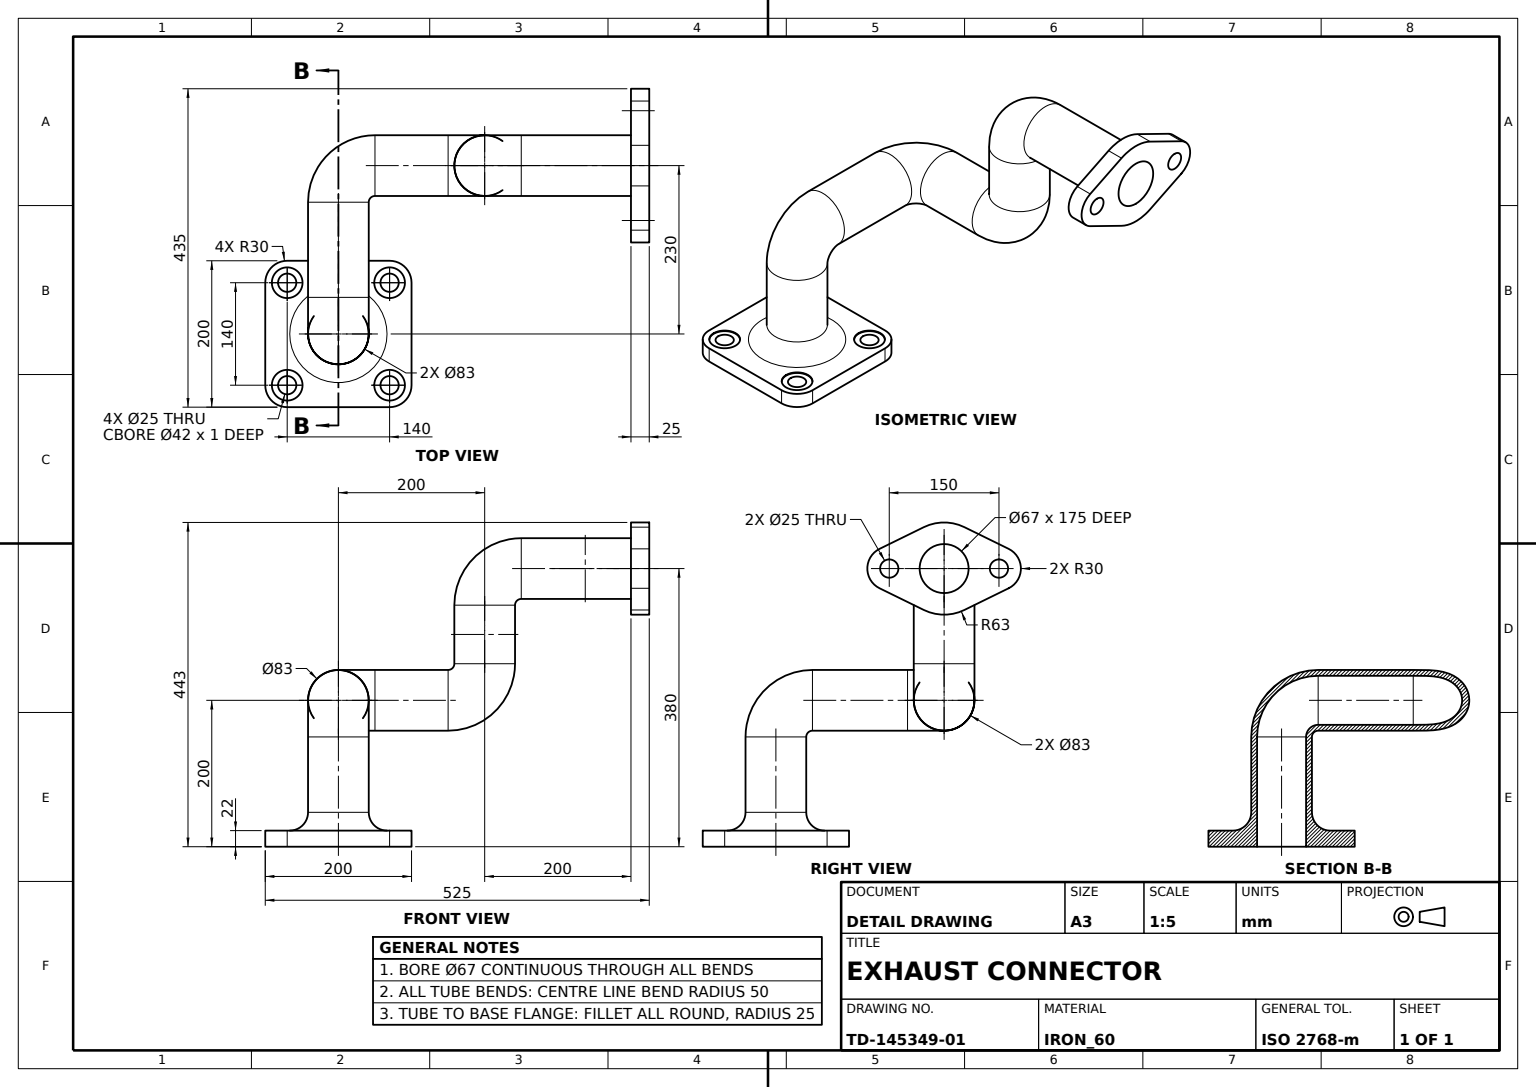
ISO-10303-21;
HEADER;
FILE_DESCRIPTION((''),'2;1');
FILE_NAME('','',(''),(''),'','','');
FILE_SCHEMA(('AUTOMOTIVE_DESIGN'));
ENDSEC;
DATA;
#1=APPLICATION_CONTEXT('');
#2=PRODUCT_CONTEXT('',#1,'mechanical');
#3=PRODUCT('','','',(#2));
#4=PRODUCT_DEFINITION_FORMATION('','',#3);
#5=PRODUCT_DEFINITION_CONTEXT('',#1,'design');
#6=PRODUCT_DEFINITION('','',#4,#5);
#7=PRODUCT_DEFINITION_SHAPE('','',#6);
#8=(LENGTH_UNIT()NAMED_UNIT(*)SI_UNIT(.MILLI.,.METRE.));
#9=(NAMED_UNIT(*)PLANE_ANGLE_UNIT()SI_UNIT($,.RADIAN.));
#10=(NAMED_UNIT(*)SI_UNIT($,.STERADIAN.)SOLID_ANGLE_UNIT());
#11=UNCERTAINTY_MEASURE_WITH_UNIT(LENGTH_MEASURE(0.005),#8,'distance_accuracy_value','');
#12=(GEOMETRIC_REPRESENTATION_CONTEXT(3)GLOBAL_UNCERTAINTY_ASSIGNED_CONTEXT((#11))GLOBAL_UNIT_ASSIGNED_CONTEXT((#8,#9,#10))REPRESENTATION_CONTEXT('',''));
#13=CARTESIAN_POINT('',(400.,202.28,323.42614));
#14=VERTEX_POINT('',#13);
#15=CARTESIAN_POINT('',(400.,257.72,323.42614));
#16=VERTEX_POINT('',#15);
#17=CARTESIAN_POINT('',(400.,230.,380.));
#18=DIRECTION('',(1.,0.,0.));
#19=DIRECTION('',(0.,1.,0.));
#20=AXIS2_PLACEMENT_3D('',#17,#18,#19);
#21=CIRCLE('',#20,63.);
#22=EDGE_CURVE('',#14,#16,#21,.T.);
#23=ORIENTED_EDGE('',*,*,#22,.T.);
#24=CARTESIAN_POINT('',(425.,257.72,323.42614));
#25=VERTEX_POINT('',#24);
#26=VECTOR('',#18,1000.);
#27=LINE('',#15,#26);
#28=EDGE_CURVE('',#16,#25,#27,.T.);
#29=ORIENTED_EDGE('',*,*,#28,.T.);
#30=CARTESIAN_POINT('',(425.,202.28,323.42614));
#31=VERTEX_POINT('',#30);
#32=CARTESIAN_POINT('',(425.,230.,380.));
#33=AXIS2_PLACEMENT_3D('',#32,#18,#19);
#34=CIRCLE('',#33,63.);
#35=EDGE_CURVE('',#31,#25,#34,.T.);
#36=ORIENTED_EDGE('',*,*,#35,.F.);
#37=LINE('',#13,#26);
#38=EDGE_CURVE('',#14,#31,#37,.T.);
#39=ORIENTED_EDGE('',*,*,#38,.F.);
#40=EDGE_LOOP('',(#23,#29,#36,#39));
#41=FACE_BOUND('',#40,.T.);
#42=DIRECTION('',(0.,0.,-1.));
#43=AXIS2_PLACEMENT_3D('',#17,#18,#42);
#44=CYLINDRICAL_SURFACE('',#43,63.);
#45=ADVANCED_FACE('',(#41),#44,.T.);
#46=CARTESIAN_POINT('',(233.5,230.,330.));
#47=VERTEX_POINT('',#46);
#48=CARTESIAN_POINT('',(200.,230.,330.));
#49=DIRECTION('',(0.,0.,1.));
#50=AXIS2_PLACEMENT_3D('',#48,#49,#18);
#51=CIRCLE('',#50,33.5);
#52=EDGE_CURVE('',#47,#47,#51,.T.);
#53=ORIENTED_EDGE('',*,*,#52,.F.);
#54=EDGE_LOOP('',(#53));
#55=FACE_BOUND('',#54,.T.);
#56=CARTESIAN_POINT('',(250.,230.,346.5));
#57=VERTEX_POINT('',#56);
#58=CARTESIAN_POINT('',(250.,230.,380.));
#59=AXIS2_PLACEMENT_3D('',#58,#18,#42);
#60=CIRCLE('',#59,33.5);
#61=EDGE_CURVE('',#57,#57,#60,.T.);
#62=ORIENTED_EDGE('',*,*,#61,.T.);
#63=EDGE_LOOP('',(#62));
#64=FACE_BOUND('',#63,.T.);
#65=CARTESIAN_POINT('',(250.,230.,330.));
#66=AXIS2_PLACEMENT_3D('',#65,#19,#49);
#67=TOROIDAL_SURFACE('',#66,50.,33.5);
#68=ADVANCED_FACE('',(#55,#64),#67,.F.);
#69=CARTESIAN_POINT('',(-82.5,-70.,21.));
#70=VERTEX_POINT('',#69);
#71=CARTESIAN_POINT('',(-70.,-70.,21.));
#72=DIRECTION('',(-1.,0.,0.));
#73=AXIS2_PLACEMENT_3D('',#71,#42,#72);
#74=CIRCLE('',#73,12.5);
#75=EDGE_CURVE('',#70,#70,#74,.F.);
#76=ORIENTED_EDGE('',*,*,#75,.F.);
#77=EDGE_LOOP('',(#76));
#78=FACE_BOUND('',#77,.T.);
#79=CARTESIAN_POINT('',(-91.,-70.,21.));
#80=VERTEX_POINT('',#79);
#81=CIRCLE('',#73,21.);
#82=EDGE_CURVE('',#80,#80,#81,.F.);
#83=ORIENTED_EDGE('',*,*,#82,.T.);
#84=EDGE_LOOP('',(#83));
#85=FACE_BOUND('',#84,.T.);
#86=PLANE('',#73);
#87=ADVANCED_FACE('',(#78,#85),#86,.F.);
#88=CARTESIAN_POINT('',(49.,70.,22.));
#89=VERTEX_POINT('',#88);
#90=CARTESIAN_POINT('',(70.,70.,22.));
#91=AXIS2_PLACEMENT_3D('',#90,#42,#72);
#92=CIRCLE('',#91,21.);
#93=EDGE_CURVE('',#89,#89,#92,.T.);
#94=ORIENTED_EDGE('',*,*,#93,.T.);
#95=EDGE_LOOP('',(#94));
#96=FACE_BOUND('',#95,.T.);
#97=CARTESIAN_POINT('',(-66.5,0.,22.));
#98=VERTEX_POINT('',#97);
#99=CARTESIAN_POINT('',(0.,0.,22.));
#100=AXIS2_PLACEMENT_3D('',#99,#42,#72);
#101=CIRCLE('',#100,66.5);
#102=EDGE_CURVE('',#98,#98,#101,.T.);
#103=ORIENTED_EDGE('',*,*,#102,.T.);
#104=EDGE_LOOP('',(#103));
#105=FACE_BOUND('',#104,.T.);
#106=CARTESIAN_POINT('',(49.,-70.,22.));
#107=VERTEX_POINT('',#106);
#108=CARTESIAN_POINT('',(70.,-70.,22.));
#109=AXIS2_PLACEMENT_3D('',#108,#42,#72);
#110=CIRCLE('',#109,21.);
#111=EDGE_CURVE('',#107,#107,#110,.T.);
#112=ORIENTED_EDGE('',*,*,#111,.T.);
#113=EDGE_LOOP('',(#112));
#114=FACE_BOUND('',#113,.T.);
#115=CARTESIAN_POINT('',(-91.,70.,22.));
#116=VERTEX_POINT('',#115);
#117=CARTESIAN_POINT('',(-70.,70.,22.));
#118=AXIS2_PLACEMENT_3D('',#117,#42,#72);
#119=CIRCLE('',#118,21.);
#120=EDGE_CURVE('',#116,#116,#119,.T.);
#121=ORIENTED_EDGE('',*,*,#120,.T.);
#122=EDGE_LOOP('',(#121));
#123=FACE_BOUND('',#122,.T.);
#124=CARTESIAN_POINT('',(100.,70.,22.));
#125=VERTEX_POINT('',#124);
#126=CARTESIAN_POINT('',(100.,-70.,22.));
#127=VERTEX_POINT('',#126);
#128=CARTESIAN_POINT('',(100.,100.,22.));
#129=DIRECTION('',(0.,-1.,0.));
#130=VECTOR('',#129,1000.);
#131=LINE('',#128,#130);
#132=EDGE_CURVE('',#125,#127,#131,.T.);
#133=ORIENTED_EDGE('',*,*,#132,.F.);
#134=CARTESIAN_POINT('',(70.,100.,22.));
#135=VERTEX_POINT('',#134);
#136=CIRCLE('',#91,30.);
#137=EDGE_CURVE('',#125,#135,#136,.F.);
#138=ORIENTED_EDGE('',*,*,#137,.T.);
#139=CARTESIAN_POINT('',(-70.,100.,22.));
#140=VERTEX_POINT('',#139);
#141=CARTESIAN_POINT('',(-100.,100.,22.));
#142=LINE('',#141,#26);
#143=EDGE_CURVE('',#140,#135,#142,.T.);
#144=ORIENTED_EDGE('',*,*,#143,.F.);
#145=CARTESIAN_POINT('',(-100.,70.,22.));
#146=VERTEX_POINT('',#145);
#147=CIRCLE('',#118,30.);
#148=EDGE_CURVE('',#140,#146,#147,.F.);
#149=ORIENTED_EDGE('',*,*,#148,.T.);
#150=CARTESIAN_POINT('',(-100.,-70.,22.));
#151=VERTEX_POINT('',#150);
#152=CARTESIAN_POINT('',(-100.,-100.,22.));
#153=VECTOR('',#19,1000.);
#154=LINE('',#152,#153);
#155=EDGE_CURVE('',#151,#146,#154,.T.);
#156=ORIENTED_EDGE('',*,*,#155,.F.);
#157=CARTESIAN_POINT('',(-70.,-100.,22.));
#158=VERTEX_POINT('',#157);
#159=CARTESIAN_POINT('',(-70.,-70.,22.));
#160=AXIS2_PLACEMENT_3D('',#159,#42,#72);
#161=CIRCLE('',#160,30.);
#162=EDGE_CURVE('',#151,#158,#161,.F.);
#163=ORIENTED_EDGE('',*,*,#162,.T.);
#164=CARTESIAN_POINT('',(70.,-100.,22.));
#165=VERTEX_POINT('',#164);
#166=CARTESIAN_POINT('',(100.,-100.,22.));
#167=VECTOR('',#72,1000.);
#168=LINE('',#166,#167);
#169=EDGE_CURVE('',#165,#158,#168,.T.);
#170=ORIENTED_EDGE('',*,*,#169,.F.);
#171=CIRCLE('',#109,30.);
#172=EDGE_CURVE('',#165,#127,#171,.F.);
#173=ORIENTED_EDGE('',*,*,#172,.T.);
#174=EDGE_LOOP('',(#133,#138,#144,#149,#156,#163,#170,#173));
#175=FACE_BOUND('',#174,.T.);
#176=CARTESIAN_POINT('',(-91.,-70.,22.));
#177=VERTEX_POINT('',#176);
#178=CIRCLE('',#160,21.);
#179=EDGE_CURVE('',#177,#177,#178,.T.);
#180=ORIENTED_EDGE('',*,*,#179,.T.);
#181=EDGE_LOOP('',(#180));
#182=FACE_BOUND('',#181,.T.);
#183=PLANE('',#100);
#184=ADVANCED_FACE('',(#96,#105,#114,#123,#175,#182),#183,.F.);
#185=CARTESIAN_POINT('',(400.,141.8,406.939933));
#186=VERTEX_POINT('',#185);
#187=CARTESIAN_POINT('',(400.,141.8,353.060067));
#188=VERTEX_POINT('',#187);
#189=CARTESIAN_POINT('',(400.,155.,380.));
#190=AXIS2_PLACEMENT_3D('',#189,#18,#19);
#191=CIRCLE('',#190,30.);
#192=EDGE_CURVE('',#186,#188,#191,.T.);
#193=ORIENTED_EDGE('',*,*,#192,.T.);
#194=CARTESIAN_POINT('',(425.,141.8,353.060067));
#195=VERTEX_POINT('',#194);
#196=LINE('',#187,#26);
#197=EDGE_CURVE('',#188,#195,#196,.T.);
#198=ORIENTED_EDGE('',*,*,#197,.T.);
#199=CARTESIAN_POINT('',(425.,141.8,406.939933));
#200=VERTEX_POINT('',#199);
#201=CARTESIAN_POINT('',(425.,155.,380.));
#202=AXIS2_PLACEMENT_3D('',#201,#18,#19);
#203=CIRCLE('',#202,30.);
#204=EDGE_CURVE('',#200,#195,#203,.T.);
#205=ORIENTED_EDGE('',*,*,#204,.F.);
#206=LINE('',#185,#26);
#207=EDGE_CURVE('',#186,#200,#206,.T.);
#208=ORIENTED_EDGE('',*,*,#207,.F.);
#209=EDGE_LOOP('',(#193,#198,#205,#208));
#210=FACE_BOUND('',#209,.T.);
#211=AXIS2_PLACEMENT_3D('',#189,#18,#42);
#212=CYLINDRICAL_SURFACE('',#211,30.);
#213=ADVANCED_FACE('',(#210),#212,.T.);
#214=CARTESIAN_POINT('',(425.,230.,413.5));
#215=VERTEX_POINT('',#214);
#216=AXIS2_PLACEMENT_3D('',#32,#72,#49);
#217=CIRCLE('',#216,33.5);
#218=EDGE_CURVE('',#215,#215,#217,.T.);
#219=ORIENTED_EDGE('',*,*,#218,.F.);
#220=EDGE_LOOP('',(#219));
#221=FACE_BOUND('',#220,.T.);
#222=ORIENTED_EDGE('',*,*,#61,.F.);
#223=EDGE_LOOP('',(#222));
#224=FACE_BOUND('',#223,.T.);
#225=CYLINDRICAL_SURFACE('',#59,33.5);
#226=ADVANCED_FACE('',(#221,#224),#225,.F.);
#227=CARTESIAN_POINT('',(49.,70.,21.));
#228=VERTEX_POINT('',#227);
#229=CARTESIAN_POINT('',(70.,70.,21.));
#230=AXIS2_PLACEMENT_3D('',#229,#42,#72);
#231=CIRCLE('',#230,21.);
#232=EDGE_CURVE('',#228,#228,#231,.F.);
#233=ORIENTED_EDGE('',*,*,#232,.F.);
#234=EDGE_LOOP('',(#233));
#235=FACE_BOUND('',#234,.T.);
#236=ORIENTED_EDGE('',*,*,#93,.F.);
#237=EDGE_LOOP('',(#236));
#238=FACE_BOUND('',#237,.T.);
#239=CYLINDRICAL_SURFACE('',#91,21.);
#240=ADVANCED_FACE('',(#235,#238),#239,.F.);
#241=CARTESIAN_POINT('',(425.,155.,392.5));
#242=VERTEX_POINT('',#241);
#243=AXIS2_PLACEMENT_3D('',#201,#72,#49);
#244=CIRCLE('',#243,12.5);
#245=EDGE_CURVE('',#242,#242,#244,.T.);
#246=ORIENTED_EDGE('',*,*,#245,.T.);
#247=EDGE_LOOP('',(#246));
#248=FACE_BOUND('',#247,.T.);
#249=CARTESIAN_POINT('',(425.,305.,392.5));
#250=VERTEX_POINT('',#249);
#251=CARTESIAN_POINT('',(425.,305.,380.));
#252=AXIS2_PLACEMENT_3D('',#251,#72,#49);
#253=CIRCLE('',#252,12.5);
#254=EDGE_CURVE('',#250,#250,#253,.T.);
#255=ORIENTED_EDGE('',*,*,#254,.T.);
#256=EDGE_LOOP('',(#255));
#257=FACE_BOUND('',#256,.T.);
#258=ORIENTED_EDGE('',*,*,#218,.T.);
#259=EDGE_LOOP('',(#258));
#260=FACE_BOUND('',#259,.T.);
#261=CARTESIAN_POINT('',(425.,318.2,353.060067));
#262=VERTEX_POINT('',#261);
#263=CARTESIAN_POINT('',(425.,318.2,406.939933));
#264=VERTEX_POINT('',#263);
#265=AXIS2_PLACEMENT_3D('',#251,#18,#19);
#266=CIRCLE('',#265,30.);
#267=EDGE_CURVE('',#262,#264,#266,.T.);
#268=ORIENTED_EDGE('',*,*,#267,.T.);
#269=CARTESIAN_POINT('',(425.,257.72,436.57386));
#270=VERTEX_POINT('',#269);
#271=DIRECTION('',(0.,-0.897997773,0.44));
#272=VECTOR('',#271,1000.);
#273=LINE('',#263,#272);
#274=EDGE_CURVE('',#264,#270,#273,.T.);
#275=ORIENTED_EDGE('',*,*,#274,.T.);
#276=CARTESIAN_POINT('',(425.,202.28,436.57386));
#277=VERTEX_POINT('',#276);
#278=EDGE_CURVE('',#270,#277,#34,.T.);
#279=ORIENTED_EDGE('',*,*,#278,.T.);
#280=DIRECTION('',(0.,-0.897997773,-0.44));
#281=VECTOR('',#280,1000.);
#282=LINE('',#276,#281);
#283=EDGE_CURVE('',#277,#200,#282,.T.);
#284=ORIENTED_EDGE('',*,*,#283,.T.);
#285=ORIENTED_EDGE('',*,*,#204,.T.);
#286=DIRECTION('',(0.,0.897997773,-0.44));
#287=VECTOR('',#286,1000.);
#288=LINE('',#194,#287);
#289=EDGE_CURVE('',#195,#31,#288,.T.);
#290=ORIENTED_EDGE('',*,*,#289,.T.);
#291=ORIENTED_EDGE('',*,*,#35,.T.);
#292=DIRECTION('',(0.,0.897997773,0.44));
#293=VECTOR('',#292,1000.);
#294=LINE('',#24,#293);
#295=EDGE_CURVE('',#25,#262,#294,.T.);
#296=ORIENTED_EDGE('',*,*,#295,.T.);
#297=EDGE_LOOP('',(#268,#275,#279,#284,#285,#290,#291,#296));
#298=FACE_BOUND('',#297,.T.);
#299=AXIS2_PLACEMENT_3D('',#251,#18,#42);
#300=PLANE('',#299);
#301=ADVANCED_FACE('',(#248,#257,#260,#298),#300,.T.);
#302=ORIENTED_EDGE('',*,*,#155,.T.);
#303=CARTESIAN_POINT('',(-100.,70.,0.));
#304=VERTEX_POINT('',#303);
#305=VECTOR('',#42,1000.);
#306=LINE('',#145,#305);
#307=EDGE_CURVE('',#146,#304,#306,.T.);
#308=ORIENTED_EDGE('',*,*,#307,.T.);
#309=CARTESIAN_POINT('',(-100.,-70.,0.));
#310=VERTEX_POINT('',#309);
#311=CARTESIAN_POINT('',(-100.,-100.,0.));
#312=LINE('',#311,#153);
#313=EDGE_CURVE('',#310,#304,#312,.T.);
#314=ORIENTED_EDGE('',*,*,#313,.F.);
#315=LINE('',#150,#305);
#316=EDGE_CURVE('',#310,#151,#315,.F.);
#317=ORIENTED_EDGE('',*,*,#316,.T.);
#318=EDGE_LOOP('',(#302,#308,#314,#317));
#319=FACE_BOUND('',#318,.T.);
#320=AXIS2_PLACEMENT_3D('',#152,#72,#49);
#321=PLANE('',#320);
#322=ADVANCED_FACE('',(#319),#321,.T.);
#323=CARTESIAN_POINT('',(233.5,230.,250.));
#324=VERTEX_POINT('',#323);
#325=CARTESIAN_POINT('',(200.,230.,250.));
#326=AXIS2_PLACEMENT_3D('',#325,#49,#18);
#327=CIRCLE('',#326,33.5);
#328=EDGE_CURVE('',#324,#324,#327,.T.);
#329=ORIENTED_EDGE('',*,*,#328,.T.);
#330=EDGE_LOOP('',(#329));
#331=FACE_BOUND('',#330,.T.);
#332=CARTESIAN_POINT('',(150.,230.,166.5));
#333=VERTEX_POINT('',#332);
#334=CARTESIAN_POINT('',(150.,230.,200.));
#335=AXIS2_PLACEMENT_3D('',#334,#18,#42);
#336=CIRCLE('',#335,33.5);
#337=EDGE_CURVE('',#333,#333,#336,.T.);
#338=ORIENTED_EDGE('',*,*,#337,.F.);
#339=EDGE_LOOP('',(#338));
#340=FACE_BOUND('',#339,.T.);
#341=CARTESIAN_POINT('',(150.,230.,250.));
#342=AXIS2_PLACEMENT_3D('',#341,#129,#42);
#343=TOROIDAL_SURFACE('',#342,50.,33.5);
#344=ADVANCED_FACE('',(#331,#340),#343,.F.);
#345=CARTESIAN_POINT('',(0.,180.,158.5));
#346=VERTEX_POINT('',#345);
#347=CARTESIAN_POINT('',(0.,180.,200.));
#348=AXIS2_PLACEMENT_3D('',#347,#129,#42);
#349=CIRCLE('',#348,41.5);
#350=EDGE_CURVE('',#346,#346,#349,.T.);
#351=ORIENTED_EDGE('',*,*,#350,.F.);
#352=EDGE_LOOP('',(#351));
#353=FACE_BOUND('',#352,.T.);
#354=CARTESIAN_POINT('',(50.,271.5,200.));
#355=VERTEX_POINT('',#354);
#356=CARTESIAN_POINT('',(50.,230.,200.));
#357=AXIS2_PLACEMENT_3D('',#356,#18,#19);
#358=CIRCLE('',#357,41.5);
#359=EDGE_CURVE('',#355,#355,#358,.T.);
#360=ORIENTED_EDGE('',*,*,#359,.F.);
#361=EDGE_LOOP('',(#360));
#362=FACE_BOUND('',#361,.T.);
#363=CARTESIAN_POINT('',(50.,180.,200.));
#364=AXIS2_PLACEMENT_3D('',#363,#42,#72);
#365=TOROIDAL_SURFACE('',#364,50.,41.5);
#366=ADVANCED_FACE('',(#353,#362),#365,.T.);
#367=CARTESIAN_POINT('',(-70.,100.,0.));
#368=VERTEX_POINT('',#367);
#369=CARTESIAN_POINT('',(-70.,70.,0.));
#370=AXIS2_PLACEMENT_3D('',#369,#42,#72);
#371=CIRCLE('',#370,30.);
#372=EDGE_CURVE('',#304,#368,#371,.T.);
#373=ORIENTED_EDGE('',*,*,#372,.F.);
#374=ORIENTED_EDGE('',*,*,#307,.F.);
#375=ORIENTED_EDGE('',*,*,#148,.F.);
#376=LINE('',#139,#305);
#377=EDGE_CURVE('',#368,#140,#376,.F.);
#378=ORIENTED_EDGE('',*,*,#377,.F.);
#379=EDGE_LOOP('',(#373,#374,#375,#378));
#380=FACE_BOUND('',#379,.T.);
#381=CYLINDRICAL_SURFACE('',#118,30.);
#382=ADVANCED_FACE('',(#380),#381,.T.);
#383=ORIENTED_EDGE('',*,*,#350,.T.);
#384=EDGE_LOOP('',(#383));
#385=FACE_BOUND('',#384,.T.);
#386=CARTESIAN_POINT('',(0.,50.,158.5));
#387=VERTEX_POINT('',#386);
#388=CARTESIAN_POINT('',(0.,50.,200.));
#389=AXIS2_PLACEMENT_3D('',#388,#129,#42);
#390=CIRCLE('',#389,41.5);
#391=EDGE_CURVE('',#387,#387,#390,.T.);
#392=ORIENTED_EDGE('',*,*,#391,.F.);
#393=EDGE_LOOP('',(#392));
#394=FACE_BOUND('',#393,.T.);
#395=AXIS2_PLACEMENT_3D('',#388,#19,#49);
#396=CYLINDRICAL_SURFACE('',#395,41.5);
#397=ADVANCED_FACE('',(#385,#394),#396,.T.);
#398=CARTESIAN_POINT('',(50.,263.5,200.));
#399=VERTEX_POINT('',#398);
#400=CIRCLE('',#357,33.5);
#401=EDGE_CURVE('',#399,#399,#400,.T.);
#402=ORIENTED_EDGE('',*,*,#401,.F.);
#403=EDGE_LOOP('',(#402));
#404=FACE_BOUND('',#403,.T.);
#405=ORIENTED_EDGE('',*,*,#337,.T.);
#406=EDGE_LOOP('',(#405));
#407=FACE_BOUND('',#406,.T.);
#408=AXIS2_PLACEMENT_3D('',#356,#18,#42);
#409=CYLINDRICAL_SURFACE('',#408,33.5);
#410=ADVANCED_FACE('',(#404,#407),#409,.F.);
#411=CARTESIAN_POINT('',(-82.5,-70.,0.));
#412=VERTEX_POINT('',#411);
#413=CARTESIAN_POINT('',(-70.,-70.,0.));
#414=AXIS2_PLACEMENT_3D('',#413,#42,#72);
#415=CIRCLE('',#414,12.5);
#416=EDGE_CURVE('',#412,#412,#415,.T.);
#417=ORIENTED_EDGE('',*,*,#416,.T.);
#418=EDGE_LOOP('',(#417));
#419=FACE_BOUND('',#418,.T.);
#420=ORIENTED_EDGE('',*,*,#75,.T.);
#421=EDGE_LOOP('',(#420));
#422=FACE_BOUND('',#421,.T.);
#423=CARTESIAN_POINT('',(-70.,-70.,-28.));
#424=AXIS2_PLACEMENT_3D('',#423,#42,#72);
#425=CYLINDRICAL_SURFACE('',#424,12.5);
#426=ADVANCED_FACE('',(#419,#422),#425,.F.);
#427=CARTESIAN_POINT('',(0.,180.,166.5));
#428=VERTEX_POINT('',#427);
#429=CIRCLE('',#348,33.5);
#430=EDGE_CURVE('',#428,#428,#429,.T.);
#431=ORIENTED_EDGE('',*,*,#430,.T.);
#432=EDGE_LOOP('',(#431));
#433=FACE_BOUND('',#432,.T.);
#434=ORIENTED_EDGE('',*,*,#401,.T.);
#435=EDGE_LOOP('',(#434));
#436=FACE_BOUND('',#435,.T.);
#437=TOROIDAL_SURFACE('',#364,50.,33.5);
#438=ADVANCED_FACE('',(#433,#436),#437,.F.);
#439=CARTESIAN_POINT('',(250.,230.,338.5));
#440=VERTEX_POINT('',#439);
#441=CIRCLE('',#59,41.5);
#442=EDGE_CURVE('',#440,#440,#441,.T.);
#443=ORIENTED_EDGE('',*,*,#442,.T.);
#444=EDGE_LOOP('',(#443));
#445=FACE_BOUND('',#444,.T.);
#446=CARTESIAN_POINT('',(400.,230.,338.5));
#447=VERTEX_POINT('',#446);
#448=CIRCLE('',#43,41.5);
#449=EDGE_CURVE('',#447,#447,#448,.T.);
#450=ORIENTED_EDGE('',*,*,#449,.F.);
#451=EDGE_LOOP('',(#450));
#452=FACE_BOUND('',#451,.T.);
#453=CYLINDRICAL_SURFACE('',#59,41.5);
#454=ADVANCED_FACE('',(#445,#452),#453,.T.);
#455=ORIENTED_EDGE('',*,*,#278,.F.);
#456=CARTESIAN_POINT('',(400.,257.72,436.57386));
#457=VERTEX_POINT('',#456);
#458=LINE('',#456,#26);
#459=EDGE_CURVE('',#457,#270,#458,.T.);
#460=ORIENTED_EDGE('',*,*,#459,.F.);
#461=CARTESIAN_POINT('',(400.,202.28,436.57386));
#462=VERTEX_POINT('',#461);
#463=EDGE_CURVE('',#457,#462,#21,.T.);
#464=ORIENTED_EDGE('',*,*,#463,.T.);
#465=LINE('',#461,#26);
#466=EDGE_CURVE('',#462,#277,#465,.T.);
#467=ORIENTED_EDGE('',*,*,#466,.T.);
#468=EDGE_LOOP('',(#455,#460,#464,#467));
#469=FACE_BOUND('',#468,.T.);
#470=ADVANCED_FACE('',(#469),#44,.T.);
#471=ORIENTED_EDGE('',*,*,#102,.F.);
#472=EDGE_LOOP('',(#471));
#473=FACE_BOUND('',#472,.T.);
#474=CARTESIAN_POINT('',(-41.5,0.,47.));
#475=VERTEX_POINT('',#474);
#476=CARTESIAN_POINT('',(0.,0.,47.));
#477=AXIS2_PLACEMENT_3D('',#476,#42,#72);
#478=CIRCLE('',#477,41.5);
#479=EDGE_CURVE('',#475,#475,#478,.F.);
#480=ORIENTED_EDGE('',*,*,#479,.F.);
#481=EDGE_LOOP('',(#480));
#482=FACE_BOUND('',#481,.T.);
#483=TOROIDAL_SURFACE('',#477,66.5,25.);
#484=ADVANCED_FACE('',(#473,#482),#483,.F.);
#485=ORIENTED_EDGE('',*,*,#479,.T.);
#486=EDGE_LOOP('',(#485));
#487=FACE_BOUND('',#486,.T.);
#488=CARTESIAN_POINT('',(0.,41.5,150.));
#489=VERTEX_POINT('',#488);
#490=CARTESIAN_POINT('',(0.,0.,150.));
#491=AXIS2_PLACEMENT_3D('',#490,#42,#19);
#492=CIRCLE('',#491,41.5);
#493=EDGE_CURVE('',#489,#489,#492,.T.);
#494=ORIENTED_EDGE('',*,*,#493,.T.);
#495=EDGE_LOOP('',(#494));
#496=FACE_BOUND('',#495,.T.);
#497=CYLINDRICAL_SURFACE('',#491,41.5);
#498=ADVANCED_FACE('',(#487,#496),#497,.T.);
#499=ORIENTED_EDGE('',*,*,#493,.F.);
#500=EDGE_LOOP('',(#499));
#501=FACE_BOUND('',#500,.T.);
#502=ORIENTED_EDGE('',*,*,#391,.T.);
#503=EDGE_LOOP('',(#502));
#504=FACE_BOUND('',#503,.T.);
#505=CARTESIAN_POINT('',(0.,50.,150.));
#506=AXIS2_PLACEMENT_3D('',#505,#18,#42);
#507=TOROIDAL_SURFACE('',#506,50.,41.5);
#508=ADVANCED_FACE('',(#501,#504),#507,.T.);
#509=ORIENTED_EDGE('',*,*,#232,.T.);
#510=EDGE_LOOP('',(#509));
#511=FACE_BOUND('',#510,.T.);
#512=CARTESIAN_POINT('',(57.5,70.,21.));
#513=VERTEX_POINT('',#512);
#514=CIRCLE('',#230,12.5);
#515=EDGE_CURVE('',#513,#513,#514,.F.);
#516=ORIENTED_EDGE('',*,*,#515,.F.);
#517=EDGE_LOOP('',(#516));
#518=FACE_BOUND('',#517,.T.);
#519=PLANE('',#230);
#520=ADVANCED_FACE('',(#511,#518),#519,.F.);
#521=ORIENTED_EDGE('',*,*,#283,.F.);
#522=ORIENTED_EDGE('',*,*,#466,.F.);
#523=LINE('',#461,#281);
#524=EDGE_CURVE('',#462,#186,#523,.T.);
#525=ORIENTED_EDGE('',*,*,#524,.T.);
#526=ORIENTED_EDGE('',*,*,#207,.T.);
#527=EDGE_LOOP('',(#521,#522,#525,#526));
#528=FACE_BOUND('',#527,.T.);
#529=DIRECTION('',(0.,-0.44,0.897997773));
#530=AXIS2_PLACEMENT_3D('',#461,#529,#280);
#531=PLANE('',#530);
#532=ADVANCED_FACE('',(#528),#531,.T.);
#533=ORIENTED_EDGE('',*,*,#111,.F.);
#534=EDGE_LOOP('',(#533));
#535=FACE_BOUND('',#534,.T.);
#536=CARTESIAN_POINT('',(49.,-70.,21.));
#537=VERTEX_POINT('',#536);
#538=CARTESIAN_POINT('',(70.,-70.,21.));
#539=AXIS2_PLACEMENT_3D('',#538,#42,#72);
#540=CIRCLE('',#539,21.);
#541=EDGE_CURVE('',#537,#537,#540,.F.);
#542=ORIENTED_EDGE('',*,*,#541,.F.);
#543=EDGE_LOOP('',(#542));
#544=FACE_BOUND('',#543,.T.);
#545=CYLINDRICAL_SURFACE('',#109,21.);
#546=ADVANCED_FACE('',(#535,#544),#545,.F.);
#547=CARTESIAN_POINT('',(0.,33.5,150.));
#548=VERTEX_POINT('',#547);
#549=CIRCLE('',#491,33.5);
#550=EDGE_CURVE('',#548,#548,#549,.T.);
#551=ORIENTED_EDGE('',*,*,#550,.F.);
#552=EDGE_LOOP('',(#551));
#553=FACE_BOUND('',#552,.T.);
#554=CARTESIAN_POINT('',(33.5,0.,0.));
#555=VERTEX_POINT('',#554);
#556=CARTESIAN_POINT('',(0.,0.,0.));
#557=AXIS2_PLACEMENT_3D('',#556,#49,#18);
#558=CIRCLE('',#557,33.5);
#559=EDGE_CURVE('',#555,#555,#558,.T.);
#560=ORIENTED_EDGE('',*,*,#559,.F.);
#561=EDGE_LOOP('',(#560));
#562=FACE_BOUND('',#561,.T.);
#563=CYLINDRICAL_SURFACE('',#491,33.5);
#564=ADVANCED_FACE('',(#553,#562),#563,.F.);
#565=CARTESIAN_POINT('',(0.,50.,166.5));
#566=VERTEX_POINT('',#565);
#567=CIRCLE('',#389,33.5);
#568=EDGE_CURVE('',#566,#566,#567,.T.);
#569=ORIENTED_EDGE('',*,*,#568,.F.);
#570=EDGE_LOOP('',(#569));
#571=FACE_BOUND('',#570,.T.);
#572=ORIENTED_EDGE('',*,*,#550,.T.);
#573=EDGE_LOOP('',(#572));
#574=FACE_BOUND('',#573,.T.);
#575=TOROIDAL_SURFACE('',#506,50.,33.5);
#576=ADVANCED_FACE('',(#571,#574),#575,.F.);
#577=CARTESIAN_POINT('',(150.,230.,158.5));
#578=VERTEX_POINT('',#577);
#579=CIRCLE('',#335,41.5);
#580=EDGE_CURVE('',#578,#578,#579,.T.);
#581=ORIENTED_EDGE('',*,*,#580,.T.);
#582=EDGE_LOOP('',(#581));
#583=FACE_BOUND('',#582,.T.);
#584=CARTESIAN_POINT('',(241.5,230.,250.));
#585=VERTEX_POINT('',#584);
#586=CIRCLE('',#326,41.5);
#587=EDGE_CURVE('',#585,#585,#586,.T.);
#588=ORIENTED_EDGE('',*,*,#587,.F.);
#589=EDGE_LOOP('',(#588));
#590=FACE_BOUND('',#589,.T.);
#591=TOROIDAL_SURFACE('',#342,50.,41.5);
#592=ADVANCED_FACE('',(#583,#590),#591,.T.);
#593=ORIENTED_EDGE('',*,*,#38,.T.);
#594=ORIENTED_EDGE('',*,*,#289,.F.);
#595=ORIENTED_EDGE('',*,*,#197,.F.);
#596=LINE('',#187,#287);
#597=EDGE_CURVE('',#188,#14,#596,.T.);
#598=ORIENTED_EDGE('',*,*,#597,.T.);
#599=EDGE_LOOP('',(#593,#594,#595,#598));
#600=FACE_BOUND('',#599,.T.);
#601=DIRECTION('',(0.,-0.44,-0.897997773));
#602=AXIS2_PLACEMENT_3D('',#187,#601,#286);
#603=PLANE('',#602);
#604=ADVANCED_FACE('',(#600),#603,.T.);
#605=ORIENTED_EDGE('',*,*,#28,.F.);
#606=CARTESIAN_POINT('',(400.,318.2,353.060067));
#607=VERTEX_POINT('',#606);
#608=LINE('',#15,#293);
#609=EDGE_CURVE('',#16,#607,#608,.T.);
#610=ORIENTED_EDGE('',*,*,#609,.T.);
#611=LINE('',#606,#26);
#612=EDGE_CURVE('',#607,#262,#611,.T.);
#613=ORIENTED_EDGE('',*,*,#612,.T.);
#614=ORIENTED_EDGE('',*,*,#295,.F.);
#615=EDGE_LOOP('',(#605,#610,#613,#614));
#616=FACE_BOUND('',#615,.T.);
#617=DIRECTION('',(0.,0.44,-0.897997773));
#618=AXIS2_PLACEMENT_3D('',#15,#617,#292);
#619=PLANE('',#618);
#620=ADVANCED_FACE('',(#616),#619,.T.);
#621=CARTESIAN_POINT('',(70.,-100.,0.));
#622=VERTEX_POINT('',#621);
#623=CARTESIAN_POINT('',(-70.,-100.,0.));
#624=VERTEX_POINT('',#623);
#625=CARTESIAN_POINT('',(100.,-100.,0.));
#626=LINE('',#625,#167);
#627=EDGE_CURVE('',#622,#624,#626,.T.);
#628=ORIENTED_EDGE('',*,*,#627,.T.);
#629=CIRCLE('',#414,30.);
#630=EDGE_CURVE('',#624,#310,#629,.T.);
#631=ORIENTED_EDGE('',*,*,#630,.T.);
#632=ORIENTED_EDGE('',*,*,#313,.T.);
#633=ORIENTED_EDGE('',*,*,#372,.T.);
#634=CARTESIAN_POINT('',(70.,100.,0.));
#635=VERTEX_POINT('',#634);
#636=CARTESIAN_POINT('',(-100.,100.,0.));
#637=LINE('',#636,#26);
#638=EDGE_CURVE('',#368,#635,#637,.T.);
#639=ORIENTED_EDGE('',*,*,#638,.T.);
#640=CARTESIAN_POINT('',(100.,70.,0.));
#641=VERTEX_POINT('',#640);
#642=CARTESIAN_POINT('',(70.,70.,0.));
#643=AXIS2_PLACEMENT_3D('',#642,#42,#72);
#644=CIRCLE('',#643,30.);
#645=EDGE_CURVE('',#635,#641,#644,.T.);
#646=ORIENTED_EDGE('',*,*,#645,.T.);
#647=CARTESIAN_POINT('',(100.,-70.,0.));
#648=VERTEX_POINT('',#647);
#649=CARTESIAN_POINT('',(100.,100.,0.));
#650=LINE('',#649,#130);
#651=EDGE_CURVE('',#641,#648,#650,.T.);
#652=ORIENTED_EDGE('',*,*,#651,.T.);
#653=CARTESIAN_POINT('',(70.,-70.,0.));
#654=AXIS2_PLACEMENT_3D('',#653,#42,#72);
#655=CIRCLE('',#654,30.);
#656=EDGE_CURVE('',#648,#622,#655,.T.);
#657=ORIENTED_EDGE('',*,*,#656,.T.);
#658=EDGE_LOOP('',(#628,#631,#632,#633,#639,#646,#652,#657));
#659=FACE_BOUND('',#658,.T.);
#660=CARTESIAN_POINT('',(57.5,-70.,0.));
#661=VERTEX_POINT('',#660);
#662=CIRCLE('',#654,12.5);
#663=EDGE_CURVE('',#661,#661,#662,.T.);
#664=ORIENTED_EDGE('',*,*,#663,.F.);
#665=EDGE_LOOP('',(#664));
#666=FACE_BOUND('',#665,.T.);
#667=CARTESIAN_POINT('',(57.5,70.,0.));
#668=VERTEX_POINT('',#667);
#669=CIRCLE('',#643,12.5);
#670=EDGE_CURVE('',#668,#668,#669,.T.);
#671=ORIENTED_EDGE('',*,*,#670,.F.);
#672=EDGE_LOOP('',(#671));
#673=FACE_BOUND('',#672,.T.);
#674=ORIENTED_EDGE('',*,*,#559,.T.);
#675=EDGE_LOOP('',(#674));
#676=FACE_BOUND('',#675,.T.);
#677=CARTESIAN_POINT('',(-82.5,70.,0.));
#678=VERTEX_POINT('',#677);
#679=CIRCLE('',#370,12.5);
#680=EDGE_CURVE('',#678,#678,#679,.T.);
#681=ORIENTED_EDGE('',*,*,#680,.F.);
#682=EDGE_LOOP('',(#681));
#683=FACE_BOUND('',#682,.T.);
#684=ORIENTED_EDGE('',*,*,#416,.F.);
#685=EDGE_LOOP('',(#684));
#686=FACE_BOUND('',#685,.T.);
#687=AXIS2_PLACEMENT_3D('',#556,#42,#72);
#688=PLANE('',#687);
#689=ADVANCED_FACE('',(#659,#666,#673,#676,#683,#686),#688,.T.);
#690=CARTESIAN_POINT('',(-91.,70.,21.));
#691=VERTEX_POINT('',#690);
#692=CARTESIAN_POINT('',(-70.,70.,21.));
#693=AXIS2_PLACEMENT_3D('',#692,#42,#72);
#694=CIRCLE('',#693,21.);
#695=EDGE_CURVE('',#691,#691,#694,.F.);
#696=ORIENTED_EDGE('',*,*,#695,.F.);
#697=EDGE_LOOP('',(#696));
#698=FACE_BOUND('',#697,.T.);
#699=ORIENTED_EDGE('',*,*,#120,.F.);
#700=EDGE_LOOP('',(#699));
#701=FACE_BOUND('',#700,.T.);
#702=CYLINDRICAL_SURFACE('',#118,21.);
#703=ADVANCED_FACE('',(#698,#701),#702,.F.);
#704=ORIENTED_EDGE('',*,*,#638,.F.);
#705=ORIENTED_EDGE('',*,*,#377,.T.);
#706=ORIENTED_EDGE('',*,*,#143,.T.);
#707=LINE('',#134,#305);
#708=EDGE_CURVE('',#135,#635,#707,.T.);
#709=ORIENTED_EDGE('',*,*,#708,.T.);
#710=EDGE_LOOP('',(#704,#705,#706,#709));
#711=FACE_BOUND('',#710,.T.);
#712=AXIS2_PLACEMENT_3D('',#141,#19,#49);
#713=PLANE('',#712);
#714=ADVANCED_FACE('',(#711),#713,.T.);
#715=ORIENTED_EDGE('',*,*,#612,.F.);
#716=CARTESIAN_POINT('',(400.,318.2,406.939933));
#717=VERTEX_POINT('',#716);
#718=CARTESIAN_POINT('',(400.,305.,380.));
#719=AXIS2_PLACEMENT_3D('',#718,#18,#19);
#720=CIRCLE('',#719,30.);
#721=EDGE_CURVE('',#607,#717,#720,.T.);
#722=ORIENTED_EDGE('',*,*,#721,.T.);
#723=LINE('',#716,#26);
#724=EDGE_CURVE('',#717,#264,#723,.T.);
#725=ORIENTED_EDGE('',*,*,#724,.T.);
#726=ORIENTED_EDGE('',*,*,#267,.F.);
#727=EDGE_LOOP('',(#715,#722,#725,#726));
#728=FACE_BOUND('',#727,.T.);
#729=AXIS2_PLACEMENT_3D('',#718,#18,#42);
#730=CYLINDRICAL_SURFACE('',#729,30.);
#731=ADVANCED_FACE('',(#728),#730,.T.);
#732=ORIENTED_EDGE('',*,*,#442,.F.);
#733=EDGE_LOOP('',(#732));
#734=FACE_BOUND('',#733,.T.);
#735=CARTESIAN_POINT('',(241.5,230.,330.));
#736=VERTEX_POINT('',#735);
#737=CIRCLE('',#50,41.5);
#738=EDGE_CURVE('',#736,#736,#737,.T.);
#739=ORIENTED_EDGE('',*,*,#738,.T.);
#740=EDGE_LOOP('',(#739));
#741=FACE_BOUND('',#740,.T.);
#742=TOROIDAL_SURFACE('',#66,50.,41.5);
#743=ADVANCED_FACE('',(#734,#741),#742,.T.);
#744=ORIENTED_EDGE('',*,*,#695,.T.);
#745=EDGE_LOOP('',(#744));
#746=FACE_BOUND('',#745,.T.);
#747=CARTESIAN_POINT('',(-82.5,70.,21.));
#748=VERTEX_POINT('',#747);
#749=CIRCLE('',#693,12.5);
#750=EDGE_CURVE('',#748,#748,#749,.F.);
#751=ORIENTED_EDGE('',*,*,#750,.F.);
#752=EDGE_LOOP('',(#751));
#753=FACE_BOUND('',#752,.T.);
#754=PLANE('',#693);
#755=ADVANCED_FACE('',(#746,#753),#754,.F.);
#756=CARTESIAN_POINT('',(400.,155.,367.5));
#757=VERTEX_POINT('',#756);
#758=CIRCLE('',#211,12.5);
#759=EDGE_CURVE('',#757,#757,#758,.T.);
#760=ORIENTED_EDGE('',*,*,#759,.F.);
#761=EDGE_LOOP('',(#760));
#762=FACE_BOUND('',#761,.T.);
#763=ORIENTED_EDGE('',*,*,#245,.F.);
#764=EDGE_LOOP('',(#763));
#765=FACE_BOUND('',#764,.T.);
#766=CYLINDRICAL_SURFACE('',#243,12.5);
#767=ADVANCED_FACE('',(#762,#765),#766,.F.);
#768=ORIENTED_EDGE('',*,*,#132,.T.);
#769=LINE('',#126,#305);
#770=EDGE_CURVE('',#127,#648,#769,.T.);
#771=ORIENTED_EDGE('',*,*,#770,.T.);
#772=ORIENTED_EDGE('',*,*,#651,.F.);
#773=LINE('',#124,#305);
#774=EDGE_CURVE('',#641,#125,#773,.F.);
#775=ORIENTED_EDGE('',*,*,#774,.T.);
#776=EDGE_LOOP('',(#768,#771,#772,#775));
#777=FACE_BOUND('',#776,.T.);
#778=AXIS2_PLACEMENT_3D('',#128,#18,#42);
#779=PLANE('',#778);
#780=ADVANCED_FACE('',(#777),#779,.T.);
#781=ORIENTED_EDGE('',*,*,#449,.T.);
#782=EDGE_LOOP('',(#781));
#783=FACE_BOUND('',#782,.T.);
#784=ORIENTED_EDGE('',*,*,#759,.T.);
#785=EDGE_LOOP('',(#784));
#786=FACE_BOUND('',#785,.T.);
#787=CARTESIAN_POINT('',(400.,305.,367.5));
#788=VERTEX_POINT('',#787);
#789=CIRCLE('',#729,12.5);
#790=EDGE_CURVE('',#788,#788,#789,.T.);
#791=ORIENTED_EDGE('',*,*,#790,.T.);
#792=EDGE_LOOP('',(#791));
#793=FACE_BOUND('',#792,.T.);
#794=ORIENTED_EDGE('',*,*,#22,.F.);
#795=ORIENTED_EDGE('',*,*,#597,.F.);
#796=ORIENTED_EDGE('',*,*,#192,.F.);
#797=ORIENTED_EDGE('',*,*,#524,.F.);
#798=ORIENTED_EDGE('',*,*,#463,.F.);
#799=LINE('',#716,#272);
#800=EDGE_CURVE('',#717,#457,#799,.T.);
#801=ORIENTED_EDGE('',*,*,#800,.F.);
#802=ORIENTED_EDGE('',*,*,#721,.F.);
#803=ORIENTED_EDGE('',*,*,#609,.F.);
#804=EDGE_LOOP('',(#794,#795,#796,#797,#798,#801,#802,#803));
#805=FACE_BOUND('',#804,.T.);
#806=PLANE('',#729);
#807=ADVANCED_FACE('',(#783,#786,#793,#805),#806,.F.);
#808=ORIENTED_EDGE('',*,*,#663,.T.);
#809=EDGE_LOOP('',(#808));
#810=FACE_BOUND('',#809,.T.);
#811=CARTESIAN_POINT('',(57.5,-70.,21.));
#812=VERTEX_POINT('',#811);
#813=CIRCLE('',#539,12.5);
#814=EDGE_CURVE('',#812,#812,#813,.F.);
#815=ORIENTED_EDGE('',*,*,#814,.T.);
#816=EDGE_LOOP('',(#815));
#817=FACE_BOUND('',#816,.T.);
#818=CARTESIAN_POINT('',(70.,-70.,-28.));
#819=AXIS2_PLACEMENT_3D('',#818,#42,#72);
#820=CYLINDRICAL_SURFACE('',#819,12.5);
#821=ADVANCED_FACE('',(#810,#817),#820,.F.);
#822=ORIENTED_EDGE('',*,*,#630,.F.);
#823=LINE('',#157,#305);
#824=EDGE_CURVE('',#158,#624,#823,.T.);
#825=ORIENTED_EDGE('',*,*,#824,.F.);
#826=ORIENTED_EDGE('',*,*,#162,.F.);
#827=ORIENTED_EDGE('',*,*,#316,.F.);
#828=EDGE_LOOP('',(#822,#825,#826,#827));
#829=FACE_BOUND('',#828,.T.);
#830=CYLINDRICAL_SURFACE('',#160,30.);
#831=ADVANCED_FACE('',(#829),#830,.T.);
#832=ORIENTED_EDGE('',*,*,#359,.T.);
#833=EDGE_LOOP('',(#832));
#834=FACE_BOUND('',#833,.T.);
#835=ORIENTED_EDGE('',*,*,#580,.F.);
#836=EDGE_LOOP('',(#835));
#837=FACE_BOUND('',#836,.T.);
#838=CYLINDRICAL_SURFACE('',#408,41.5);
#839=ADVANCED_FACE('',(#834,#837),#838,.T.);
#840=ORIENTED_EDGE('',*,*,#568,.T.);
#841=EDGE_LOOP('',(#840));
#842=FACE_BOUND('',#841,.T.);
#843=ORIENTED_EDGE('',*,*,#430,.F.);
#844=EDGE_LOOP('',(#843));
#845=FACE_BOUND('',#844,.T.);
#846=CYLINDRICAL_SURFACE('',#395,33.5);
#847=ADVANCED_FACE('',(#842,#845),#846,.F.);
#848=ORIENTED_EDGE('',*,*,#254,.F.);
#849=EDGE_LOOP('',(#848));
#850=FACE_BOUND('',#849,.T.);
#851=ORIENTED_EDGE('',*,*,#790,.F.);
#852=EDGE_LOOP('',(#851));
#853=FACE_BOUND('',#852,.T.);
#854=CYLINDRICAL_SURFACE('',#252,12.5);
#855=ADVANCED_FACE('',(#850,#853),#854,.F.);
#856=ORIENTED_EDGE('',*,*,#680,.T.);
#857=EDGE_LOOP('',(#856));
#858=FACE_BOUND('',#857,.T.);
#859=ORIENTED_EDGE('',*,*,#750,.T.);
#860=EDGE_LOOP('',(#859));
#861=FACE_BOUND('',#860,.T.);
#862=CARTESIAN_POINT('',(-70.,70.,-28.));
#863=AXIS2_PLACEMENT_3D('',#862,#42,#72);
#864=CYLINDRICAL_SURFACE('',#863,12.5);
#865=ADVANCED_FACE('',(#858,#861),#864,.F.);
#866=ORIENTED_EDGE('',*,*,#724,.F.);
#867=ORIENTED_EDGE('',*,*,#800,.T.);
#868=ORIENTED_EDGE('',*,*,#459,.T.);
#869=ORIENTED_EDGE('',*,*,#274,.F.);
#870=EDGE_LOOP('',(#866,#867,#868,#869));
#871=FACE_BOUND('',#870,.T.);
#872=DIRECTION('',(0.,0.44,0.897997773));
#873=AXIS2_PLACEMENT_3D('',#716,#872,#271);
#874=PLANE('',#873);
#875=ADVANCED_FACE('',(#871),#874,.T.);
#876=LINE('',#164,#305);
#877=EDGE_CURVE('',#622,#165,#876,.F.);
#878=ORIENTED_EDGE('',*,*,#877,.T.);
#879=ORIENTED_EDGE('',*,*,#169,.T.);
#880=ORIENTED_EDGE('',*,*,#824,.T.);
#881=ORIENTED_EDGE('',*,*,#627,.F.);
#882=EDGE_LOOP('',(#878,#879,#880,#881));
#883=FACE_BOUND('',#882,.T.);
#884=AXIS2_PLACEMENT_3D('',#166,#129,#42);
#885=PLANE('',#884);
#886=ADVANCED_FACE('',(#883),#885,.T.);
#887=ORIENTED_EDGE('',*,*,#587,.T.);
#888=EDGE_LOOP('',(#887));
#889=FACE_BOUND('',#888,.T.);
#890=ORIENTED_EDGE('',*,*,#738,.F.);
#891=EDGE_LOOP('',(#890));
#892=FACE_BOUND('',#891,.T.);
#893=CYLINDRICAL_SURFACE('',#326,41.5);
#894=ADVANCED_FACE('',(#889,#892),#893,.T.);
#895=ORIENTED_EDGE('',*,*,#670,.T.);
#896=EDGE_LOOP('',(#895));
#897=FACE_BOUND('',#896,.T.);
#898=ORIENTED_EDGE('',*,*,#515,.T.);
#899=EDGE_LOOP('',(#898));
#900=FACE_BOUND('',#899,.T.);
#901=CARTESIAN_POINT('',(70.,70.,-28.));
#902=AXIS2_PLACEMENT_3D('',#901,#42,#72);
#903=CYLINDRICAL_SURFACE('',#902,12.5);
#904=ADVANCED_FACE('',(#897,#900),#903,.F.);
#905=ORIENTED_EDGE('',*,*,#645,.F.);
#906=ORIENTED_EDGE('',*,*,#708,.F.);
#907=ORIENTED_EDGE('',*,*,#137,.F.);
#908=ORIENTED_EDGE('',*,*,#774,.F.);
#909=EDGE_LOOP('',(#905,#906,#907,#908));
#910=FACE_BOUND('',#909,.T.);
#911=CYLINDRICAL_SURFACE('',#91,30.);
#912=ADVANCED_FACE('',(#910),#911,.T.);
#913=ORIENTED_EDGE('',*,*,#877,.F.);
#914=ORIENTED_EDGE('',*,*,#656,.F.);
#915=ORIENTED_EDGE('',*,*,#770,.F.);
#916=ORIENTED_EDGE('',*,*,#172,.F.);
#917=EDGE_LOOP('',(#913,#914,#915,#916));
#918=FACE_BOUND('',#917,.T.);
#919=CYLINDRICAL_SURFACE('',#109,30.);
#920=ADVANCED_FACE('',(#918),#919,.T.);
#921=ORIENTED_EDGE('',*,*,#179,.F.);
#922=EDGE_LOOP('',(#921));
#923=FACE_BOUND('',#922,.T.);
#924=ORIENTED_EDGE('',*,*,#82,.F.);
#925=EDGE_LOOP('',(#924));
#926=FACE_BOUND('',#925,.T.);
#927=CYLINDRICAL_SURFACE('',#160,21.);
#928=ADVANCED_FACE('',(#923,#926),#927,.F.);
#929=ORIENTED_EDGE('',*,*,#541,.T.);
#930=EDGE_LOOP('',(#929));
#931=FACE_BOUND('',#930,.T.);
#932=ORIENTED_EDGE('',*,*,#814,.F.);
#933=EDGE_LOOP('',(#932));
#934=FACE_BOUND('',#933,.T.);
#935=PLANE('',#539);
#936=ADVANCED_FACE('',(#931,#934),#935,.F.);
#937=ORIENTED_EDGE('',*,*,#52,.T.);
#938=EDGE_LOOP('',(#937));
#939=FACE_BOUND('',#938,.T.);
#940=ORIENTED_EDGE('',*,*,#328,.F.);
#941=EDGE_LOOP('',(#940));
#942=FACE_BOUND('',#941,.T.);
#943=CYLINDRICAL_SURFACE('',#326,33.5);
#944=ADVANCED_FACE('',(#939,#942),#943,.F.);
#945=CLOSED_SHELL('',(#45,#68,#87,#184,#213,#226,#240,#301,#322,#344,#366,#382,#397,#410,#426,#438,#454,#470,#484,#498,#508,#520,#532,#546,#564,#576,#592,#604,#620,#689,#703,#714,#731,#743,#755,#767,#780,#807,#821,#831,#839,#847,#855,#865,#875,#886,#894,#904,#912,#920,#928,#936,#944));
#946=MANIFOLD_SOLID_BREP('',#945);
#947=ADVANCED_BREP_SHAPE_REPRESENTATION('',(#946),#12);
#948=SHAPE_DEFINITION_REPRESENTATION(#7,#947);
ENDSEC;
END-ISO-10303-21;
